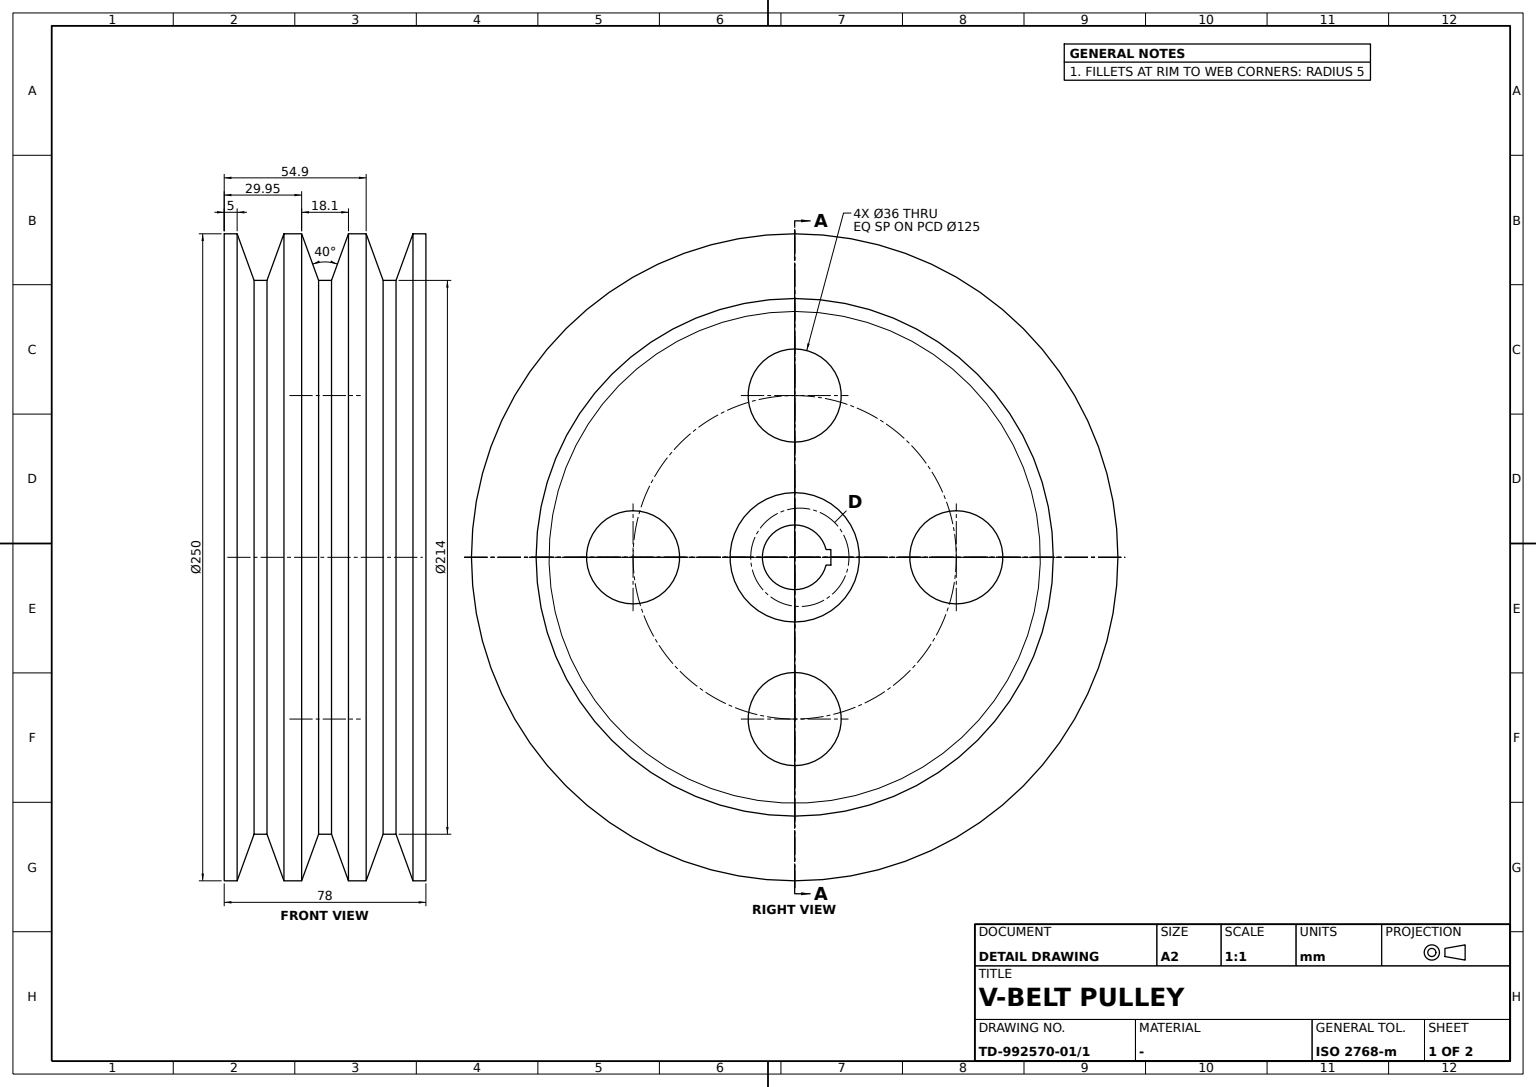
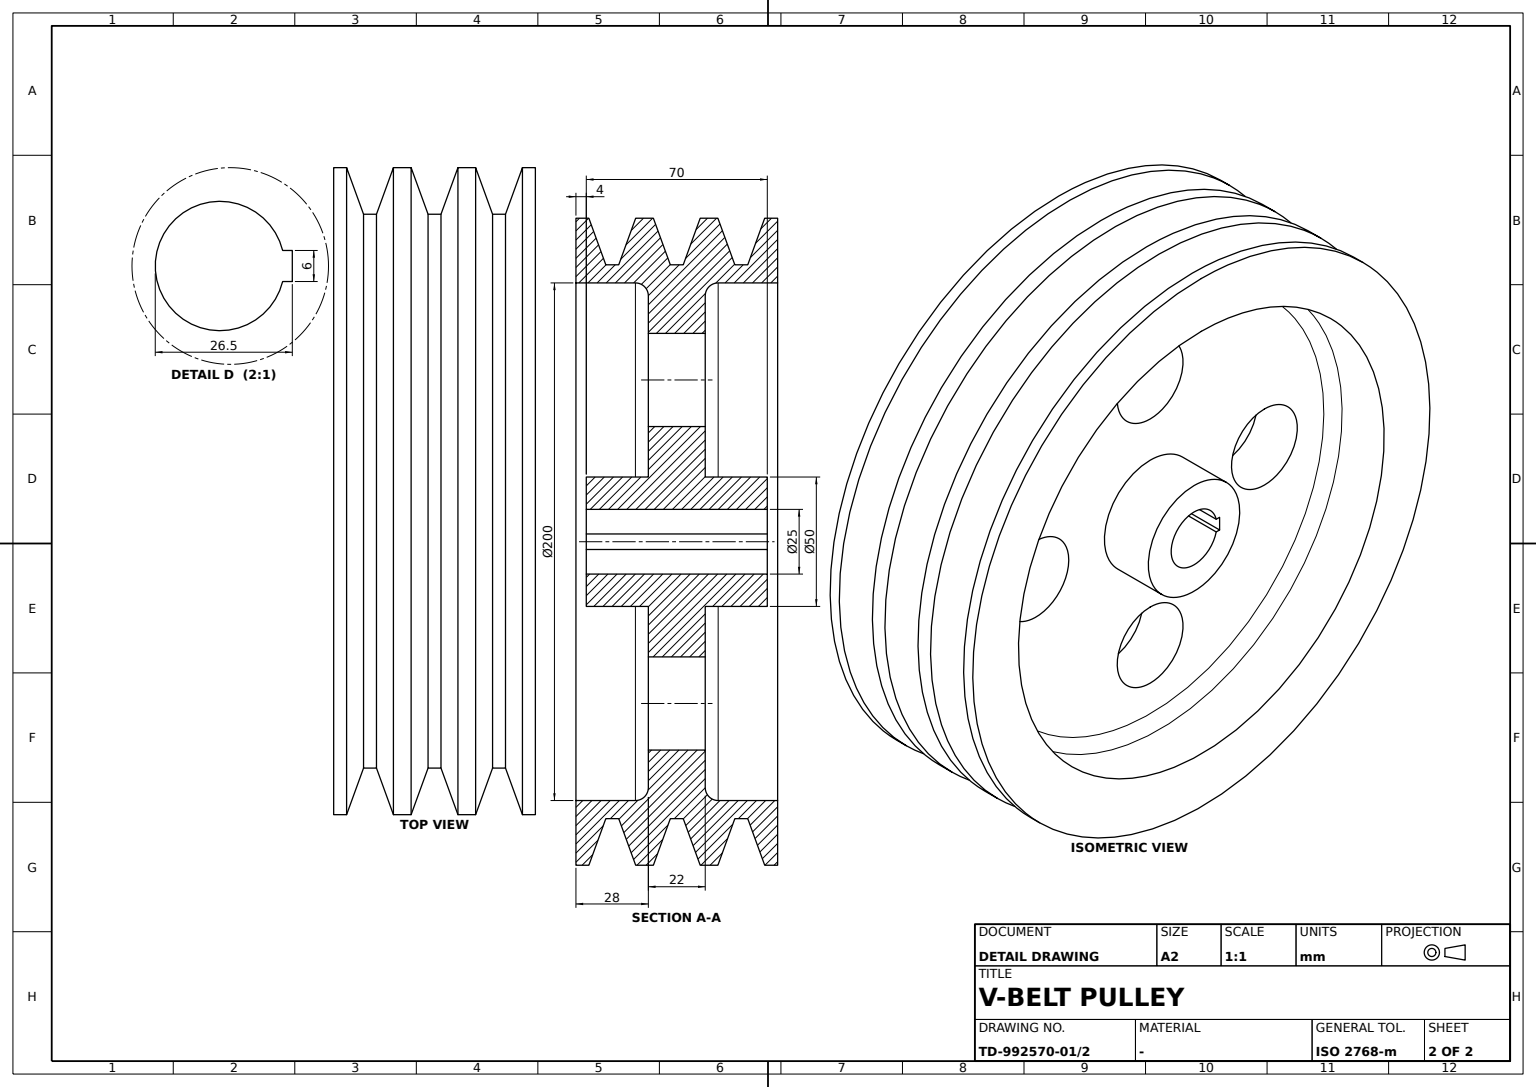
ISO-10303-21;
HEADER;
FILE_DESCRIPTION((''),'2;1');
FILE_NAME('','',(''),(''),'','','');
FILE_SCHEMA(('AUTOMOTIVE_DESIGN'));
ENDSEC;
DATA;
#1=APPLICATION_CONTEXT('');
#2=PRODUCT_CONTEXT('',#1,'mechanical');
#3=PRODUCT('','','',(#2));
#4=PRODUCT_DEFINITION_FORMATION('','',#3);
#5=PRODUCT_DEFINITION_CONTEXT('',#1,'design');
#6=PRODUCT_DEFINITION('','',#4,#5);
#7=PRODUCT_DEFINITION_SHAPE('','',#6);
#8=(LENGTH_UNIT()NAMED_UNIT(*)SI_UNIT(.MILLI.,.METRE.));
#9=(NAMED_UNIT(*)PLANE_ANGLE_UNIT()SI_UNIT($,.RADIAN.));
#10=(NAMED_UNIT(*)SI_UNIT($,.STERADIAN.)SOLID_ANGLE_UNIT());
#11=UNCERTAINTY_MEASURE_WITH_UNIT(LENGTH_MEASURE(0.005),#8,'distance_accuracy_value','');
#12=(GEOMETRIC_REPRESENTATION_CONTEXT(3)GLOBAL_UNCERTAINTY_ASSIGNED_CONTEXT((#11))GLOBAL_UNIT_ASSIGNED_CONTEXT((#8,#9,#10))REPRESENTATION_CONTEXT('',''));
#13=CARTESIAN_POINT('',(0.,27.448536,107.));
#14=VERTEX_POINT('',#13);
#15=CARTESIAN_POINT('',(0.,27.448536,0.));
#16=DIRECTION('',(0.,1.,0.));
#17=DIRECTION('',(0.,0.,1.));
#18=AXIS2_PLACEMENT_3D('',#15,#16,#17);
#19=CIRCLE('',#18,107.);
#20=EDGE_CURVE('',#14,#14,#19,.T.);
#21=ORIENTED_EDGE('',*,*,#20,.T.);
#22=EDGE_LOOP('',(#21));
#23=FACE_BOUND('',#22,.T.);
#24=CARTESIAN_POINT('',(0.,34.,125.));
#25=VERTEX_POINT('',#24);
#26=CARTESIAN_POINT('',(0.,34.,0.));
#27=AXIS2_PLACEMENT_3D('',#26,#16,#17);
#28=CIRCLE('',#27,125.);
#29=EDGE_CURVE('',#25,#25,#28,.T.);
#30=ORIENTED_EDGE('',*,*,#29,.F.);
#31=EDGE_LOOP('',(#30));
#32=FACE_BOUND('',#31,.T.);
#33=DIRECTION('',(1.,0.,0.));
#34=AXIS2_PLACEMENT_3D('',#15,#16,#33);
#35=CONICAL_SURFACE('',#34,107.,1.221730476);
#36=ADVANCED_FACE('',(#23,#32),#35,.T.);
#37=CARTESIAN_POINT('',(0.,-15.897072,125.));
#38=VERTEX_POINT('',#37);
#39=CARTESIAN_POINT('',(0.,-15.897072,0.));
#40=AXIS2_PLACEMENT_3D('',#39,#16,#17);
#41=CIRCLE('',#40,125.);
#42=EDGE_CURVE('',#38,#38,#41,.T.);
#43=ORIENTED_EDGE('',*,*,#42,.F.);
#44=EDGE_LOOP('',(#43));
#45=FACE_BOUND('',#44,.T.);
#46=CARTESIAN_POINT('',(0.,-22.448536,107.));
#47=VERTEX_POINT('',#46);
#48=CARTESIAN_POINT('',(0.,-22.448536,0.));
#49=AXIS2_PLACEMENT_3D('',#48,#16,#17);
#50=CIRCLE('',#49,107.);
#51=EDGE_CURVE('',#47,#47,#50,.T.);
#52=ORIENTED_EDGE('',*,*,#51,.T.);
#53=EDGE_LOOP('',(#52));
#54=FACE_BOUND('',#53,.T.);
#55=AXIS2_PLACEMENT_3D('',#48,#16,#33);
#56=CONICAL_SURFACE('',#55,107.,1.221730476);
#57=ADVANCED_FACE('',(#45,#54),#56,.T.);
#58=CARTESIAN_POINT('',(0.,-2.5,-107.));
#59=VERTEX_POINT('',#58);
#60=CARTESIAN_POINT('',(0.,-2.5,0.));
#61=DIRECTION('',(0.,-1.,0.));
#62=DIRECTION('',(0.,0.,-1.));
#63=AXIS2_PLACEMENT_3D('',#60,#61,#62);
#64=CIRCLE('',#63,107.);
#65=EDGE_CURVE('',#59,#59,#64,.F.);
#66=ORIENTED_EDGE('',*,*,#65,.T.);
#67=EDGE_LOOP('',(#66));
#68=FACE_BOUND('',#67,.T.);
#69=CARTESIAN_POINT('',(0.,2.5,107.));
#70=VERTEX_POINT('',#69);
#71=CARTESIAN_POINT('',(0.,2.5,0.));
#72=AXIS2_PLACEMENT_3D('',#71,#16,#17);
#73=CIRCLE('',#72,107.);
#74=EDGE_CURVE('',#70,#70,#73,.T.);
#75=ORIENTED_EDGE('',*,*,#74,.F.);
#76=EDGE_LOOP('',(#75));
#77=FACE_BOUND('',#76,.T.);
#78=CARTESIAN_POINT('',(0.,0.,0.));
#79=AXIS2_PLACEMENT_3D('',#78,#16,#33);
#80=CYLINDRICAL_SURFACE('',#79,107.);
#81=ADVANCED_FACE('',(#68,#77),#80,.T.);
#82=CARTESIAN_POINT('',(0.,39.,100.));
#83=VERTEX_POINT('',#82);
#84=CARTESIAN_POINT('',(0.,39.,0.));
#85=AXIS2_PLACEMENT_3D('',#84,#16,#17);
#86=CIRCLE('',#85,100.);
#87=EDGE_CURVE('',#83,#83,#86,.T.);
#88=ORIENTED_EDGE('',*,*,#87,.T.);
#89=EDGE_LOOP('',(#88));
#90=FACE_BOUND('',#89,.T.);
#91=CARTESIAN_POINT('',(0.,16.,100.));
#92=VERTEX_POINT('',#91);
#93=CARTESIAN_POINT('',(0.,16.,0.));
#94=AXIS2_PLACEMENT_3D('',#93,#16,#17);
#95=CIRCLE('',#94,100.);
#96=EDGE_CURVE('',#92,#92,#95,.T.);
#97=ORIENTED_EDGE('',*,*,#96,.F.);
#98=EDGE_LOOP('',(#97));
#99=FACE_BOUND('',#98,.T.);
#100=CYLINDRICAL_SURFACE('',#79,100.);
#101=ADVANCED_FACE('',(#90,#99),#100,.F.);
#102=CARTESIAN_POINT('',(0.,35.,25.));
#103=VERTEX_POINT('',#102);
#104=CARTESIAN_POINT('',(0.,35.,0.));
#105=AXIS2_PLACEMENT_3D('',#104,#16,#17);
#106=CIRCLE('',#105,25.);
#107=EDGE_CURVE('',#103,#103,#106,.T.);
#108=ORIENTED_EDGE('',*,*,#107,.F.);
#109=EDGE_LOOP('',(#108));
#110=FACE_BOUND('',#109,.T.);
#111=CARTESIAN_POINT('',(0.,11.,25.));
#112=VERTEX_POINT('',#111);
#113=CARTESIAN_POINT('',(0.,11.,0.));
#114=AXIS2_PLACEMENT_3D('',#113,#16,#17);
#115=CIRCLE('',#114,25.);
#116=EDGE_CURVE('',#112,#112,#115,.T.);
#117=ORIENTED_EDGE('',*,*,#116,.T.);
#118=EDGE_LOOP('',(#117));
#119=FACE_BOUND('',#118,.T.);
#120=CYLINDRICAL_SURFACE('',#79,25.);
#121=ADVANCED_FACE('',(#110,#119),#120,.T.);
#122=CARTESIAN_POINT('',(0.,-11.,-44.5));
#123=VERTEX_POINT('',#122);
#124=CARTESIAN_POINT('',(0.,-11.,-62.5));
#125=AXIS2_PLACEMENT_3D('',#124,#16,#17);
#126=CIRCLE('',#125,18.);
#127=EDGE_CURVE('',#123,#123,#126,.T.);
#128=ORIENTED_EDGE('',*,*,#127,.T.);
#129=EDGE_LOOP('',(#128));
#130=FACE_BOUND('',#129,.T.);
#131=CARTESIAN_POINT('',(0.,-11.,25.));
#132=VERTEX_POINT('',#131);
#133=CARTESIAN_POINT('',(0.,-11.,0.));
#134=AXIS2_PLACEMENT_3D('',#133,#16,#17);
#135=CIRCLE('',#134,25.);
#136=EDGE_CURVE('',#132,#132,#135,.T.);
#137=ORIENTED_EDGE('',*,*,#136,.T.);
#138=EDGE_LOOP('',(#137));
#139=FACE_BOUND('',#138,.T.);
#140=CARTESIAN_POINT('',(0.,-11.,95.));
#141=VERTEX_POINT('',#140);
#142=CIRCLE('',#134,95.);
#143=EDGE_CURVE('',#141,#141,#142,.T.);
#144=ORIENTED_EDGE('',*,*,#143,.F.);
#145=EDGE_LOOP('',(#144));
#146=FACE_BOUND('',#145,.T.);
#147=CARTESIAN_POINT('',(0.,-11.,80.5));
#148=VERTEX_POINT('',#147);
#149=CARTESIAN_POINT('',(0.,-11.,62.5));
#150=AXIS2_PLACEMENT_3D('',#149,#16,#17);
#151=CIRCLE('',#150,18.);
#152=EDGE_CURVE('',#148,#148,#151,.T.);
#153=ORIENTED_EDGE('',*,*,#152,.T.);
#154=EDGE_LOOP('',(#153));
#155=FACE_BOUND('',#154,.T.);
#156=CARTESIAN_POINT('',(62.5,-11.,18.));
#157=VERTEX_POINT('',#156);
#158=CARTESIAN_POINT('',(62.5,-11.,0.));
#159=AXIS2_PLACEMENT_3D('',#158,#16,#17);
#160=CIRCLE('',#159,18.);
#161=EDGE_CURVE('',#157,#157,#160,.T.);
#162=ORIENTED_EDGE('',*,*,#161,.T.);
#163=EDGE_LOOP('',(#162));
#164=FACE_BOUND('',#163,.T.);
#165=CARTESIAN_POINT('',(-62.5,-11.,18.));
#166=VERTEX_POINT('',#165);
#167=CARTESIAN_POINT('',(-62.5,-11.,0.));
#168=AXIS2_PLACEMENT_3D('',#167,#16,#17);
#169=CIRCLE('',#168,18.);
#170=EDGE_CURVE('',#166,#166,#169,.T.);
#171=ORIENTED_EDGE('',*,*,#170,.T.);
#172=EDGE_LOOP('',(#171));
#173=FACE_BOUND('',#172,.T.);
#174=CARTESIAN_POINT('',(0.,-11.,100.));
#175=AXIS2_PLACEMENT_3D('',#174,#16,#33);
#176=PLANE('',#175);
#177=ADVANCED_FACE('',(#130,#139,#146,#155,#164,#173),#176,.F.);
#178=CARTESIAN_POINT('',(0.,39.,125.));
#179=VERTEX_POINT('',#178);
#180=CIRCLE('',#85,125.);
#181=EDGE_CURVE('',#179,#179,#180,.T.);
#182=ORIENTED_EDGE('',*,*,#181,.F.);
#183=EDGE_LOOP('',(#182));
#184=FACE_BOUND('',#183,.T.);
#185=ORIENTED_EDGE('',*,*,#29,.T.);
#186=EDGE_LOOP('',(#185));
#187=FACE_BOUND('',#186,.T.);
#188=CYLINDRICAL_SURFACE('',#79,125.);
#189=ADVANCED_FACE('',(#184,#187),#188,.T.);
#190=CARTESIAN_POINT('',(-14.,35.,-3.));
#191=VERTEX_POINT('',#190);
#192=CARTESIAN_POINT('',(-14.,-35.,-3.));
#193=VERTEX_POINT('',#192);
#194=VECTOR('',#61,1000.);
#195=LINE('',#190,#194);
#196=EDGE_CURVE('',#191,#193,#195,.T.);
#197=ORIENTED_EDGE('',*,*,#196,.T.);
#198=CARTESIAN_POINT('',(-12.134661,-35.,-3.));
#199=VERTEX_POINT('',#198);
#200=VECTOR('',#33,1000.);
#201=LINE('',#192,#200);
#202=EDGE_CURVE('',#193,#199,#201,.T.);
#203=ORIENTED_EDGE('',*,*,#202,.T.);
#204=CARTESIAN_POINT('',(-12.134661,35.,-3.));
#205=VERTEX_POINT('',#204);
#206=VECTOR('',#16,1000.);
#207=LINE('',#204,#206);
#208=EDGE_CURVE('',#205,#199,#207,.F.);
#209=ORIENTED_EDGE('',*,*,#208,.F.);
#210=LINE('',#190,#200);
#211=EDGE_CURVE('',#191,#205,#210,.T.);
#212=ORIENTED_EDGE('',*,*,#211,.F.);
#213=EDGE_LOOP('',(#197,#203,#209,#212));
#214=FACE_BOUND('',#213,.T.);
#215=AXIS2_PLACEMENT_3D('',#190,#62,#33);
#216=PLANE('',#215);
#217=ADVANCED_FACE('',(#214),#216,.F.);
#218=CARTESIAN_POINT('',(0.,9.051464,125.));
#219=VERTEX_POINT('',#218);
#220=CARTESIAN_POINT('',(0.,9.051464,0.));
#221=AXIS2_PLACEMENT_3D('',#220,#16,#17);
#222=CIRCLE('',#221,125.);
#223=EDGE_CURVE('',#219,#219,#222,.T.);
#224=ORIENTED_EDGE('',*,*,#223,.T.);
#225=EDGE_LOOP('',(#224));
#226=FACE_BOUND('',#225,.T.);
#227=CARTESIAN_POINT('',(0.,15.897072,-125.));
#228=VERTEX_POINT('',#227);
#229=CARTESIAN_POINT('',(0.,15.897072,0.));
#230=AXIS2_PLACEMENT_3D('',#229,#61,#62);
#231=CIRCLE('',#230,125.);
#232=EDGE_CURVE('',#228,#228,#231,.F.);
#233=ORIENTED_EDGE('',*,*,#232,.F.);
#234=EDGE_LOOP('',(#233));
#235=FACE_BOUND('',#234,.T.);
#236=ADVANCED_FACE('',(#226,#235),#188,.T.);
#237=CARTESIAN_POINT('',(0.,11.,95.));
#238=VERTEX_POINT('',#237);
#239=CIRCLE('',#114,95.);
#240=EDGE_CURVE('',#238,#238,#239,.T.);
#241=ORIENTED_EDGE('',*,*,#240,.T.);
#242=EDGE_LOOP('',(#241));
#243=FACE_BOUND('',#242,.T.);
#244=CARTESIAN_POINT('',(0.,11.,-44.5));
#245=VERTEX_POINT('',#244);
#246=CARTESIAN_POINT('',(0.,11.,-62.5));
#247=AXIS2_PLACEMENT_3D('',#246,#16,#17);
#248=CIRCLE('',#247,18.);
#249=EDGE_CURVE('',#245,#245,#248,.T.);
#250=ORIENTED_EDGE('',*,*,#249,.F.);
#251=EDGE_LOOP('',(#250));
#252=FACE_BOUND('',#251,.T.);
#253=CARTESIAN_POINT('',(-62.5,11.,18.));
#254=VERTEX_POINT('',#253);
#255=CARTESIAN_POINT('',(-62.5,11.,0.));
#256=AXIS2_PLACEMENT_3D('',#255,#16,#17);
#257=CIRCLE('',#256,18.);
#258=EDGE_CURVE('',#254,#254,#257,.T.);
#259=ORIENTED_EDGE('',*,*,#258,.F.);
#260=EDGE_LOOP('',(#259));
#261=FACE_BOUND('',#260,.T.);
#262=CARTESIAN_POINT('',(62.5,11.,18.));
#263=VERTEX_POINT('',#262);
#264=CARTESIAN_POINT('',(62.5,11.,0.));
#265=AXIS2_PLACEMENT_3D('',#264,#16,#17);
#266=CIRCLE('',#265,18.);
#267=EDGE_CURVE('',#263,#263,#266,.T.);
#268=ORIENTED_EDGE('',*,*,#267,.F.);
#269=EDGE_LOOP('',(#268));
#270=FACE_BOUND('',#269,.T.);
#271=CARTESIAN_POINT('',(0.,11.,80.5));
#272=VERTEX_POINT('',#271);
#273=CARTESIAN_POINT('',(0.,11.,62.5));
#274=AXIS2_PLACEMENT_3D('',#273,#16,#17);
#275=CIRCLE('',#274,18.);
#276=EDGE_CURVE('',#272,#272,#275,.T.);
#277=ORIENTED_EDGE('',*,*,#276,.F.);
#278=EDGE_LOOP('',(#277));
#279=FACE_BOUND('',#278,.T.);
#280=ORIENTED_EDGE('',*,*,#116,.F.);
#281=EDGE_LOOP('',(#280));
#282=FACE_BOUND('',#281,.T.);
#283=CARTESIAN_POINT('',(0.,11.,100.));
#284=AXIS2_PLACEMENT_3D('',#283,#16,#33);
#285=PLANE('',#284);
#286=ADVANCED_FACE('',(#243,#252,#261,#270,#279,#282),#285,.T.);
#287=ORIENTED_EDGE('',*,*,#65,.F.);
#288=EDGE_LOOP('',(#287));
#289=FACE_BOUND('',#288,.T.);
#290=CARTESIAN_POINT('',(0.,-9.051464,-125.));
#291=VERTEX_POINT('',#290);
#292=CARTESIAN_POINT('',(0.,-9.051464,0.));
#293=AXIS2_PLACEMENT_3D('',#292,#61,#62);
#294=CIRCLE('',#293,125.);
#295=EDGE_CURVE('',#291,#291,#294,.F.);
#296=ORIENTED_EDGE('',*,*,#295,.T.);
#297=EDGE_LOOP('',(#296));
#298=FACE_BOUND('',#297,.T.);
#299=AXIS2_PLACEMENT_3D('',#60,#61,#33);
#300=CONICAL_SURFACE('',#299,107.,1.221730476);
#301=ADVANCED_FACE('',(#289,#298),#300,.T.);
#302=CARTESIAN_POINT('',(0.,-35.,25.));
#303=VERTEX_POINT('',#302);
#304=CARTESIAN_POINT('',(0.,-35.,0.));
#305=AXIS2_PLACEMENT_3D('',#304,#16,#17);
#306=CIRCLE('',#305,25.);
#307=EDGE_CURVE('',#303,#303,#306,.T.);
#308=ORIENTED_EDGE('',*,*,#307,.F.);
#309=EDGE_LOOP('',(#308));
#310=FACE_BOUND('',#309,.T.);
#311=CARTESIAN_POINT('',(-12.134661,-35.,3.));
#312=VERTEX_POINT('',#311);
#313=CARTESIAN_POINT('',(-14.,-35.,3.));
#314=VERTEX_POINT('',#313);
#315=DIRECTION('',(-1.,0.,0.));
#316=VECTOR('',#315,1000.);
#317=LINE('',#311,#316);
#318=EDGE_CURVE('',#312,#314,#317,.T.);
#319=ORIENTED_EDGE('',*,*,#318,.F.);
#320=CIRCLE('',#305,12.5);
#321=EDGE_CURVE('',#312,#199,#320,.T.);
#322=ORIENTED_EDGE('',*,*,#321,.T.);
#323=ORIENTED_EDGE('',*,*,#202,.F.);
#324=VECTOR('',#62,1000.);
#325=LINE('',#313,#324);
#326=EDGE_CURVE('',#314,#193,#325,.T.);
#327=ORIENTED_EDGE('',*,*,#326,.F.);
#328=EDGE_LOOP('',(#319,#322,#323,#327));
#329=FACE_BOUND('',#328,.T.);
#330=AXIS2_PLACEMENT_3D('',#302,#16,#33);
#331=PLANE('',#330);
#332=ADVANCED_FACE('',(#310,#329),#331,.F.);
#333=ORIENTED_EDGE('',*,*,#170,.F.);
#334=EDGE_LOOP('',(#333));
#335=FACE_BOUND('',#334,.T.);
#336=ORIENTED_EDGE('',*,*,#258,.T.);
#337=EDGE_LOOP('',(#336));
#338=FACE_BOUND('',#337,.T.);
#339=CARTESIAN_POINT('',(-62.5,-1.,0.));
#340=AXIS2_PLACEMENT_3D('',#339,#16,#315);
#341=CYLINDRICAL_SURFACE('',#340,18.);
#342=ADVANCED_FACE('',(#335,#338),#341,.F.);
#343=CARTESIAN_POINT('',(0.,-34.,-125.));
#344=VERTEX_POINT('',#343);
#345=CARTESIAN_POINT('',(0.,-34.,0.));
#346=AXIS2_PLACEMENT_3D('',#345,#61,#62);
#347=CIRCLE('',#346,125.);
#348=EDGE_CURVE('',#344,#344,#347,.F.);
#349=ORIENTED_EDGE('',*,*,#348,.T.);
#350=EDGE_LOOP('',(#349));
#351=FACE_BOUND('',#350,.T.);
#352=CARTESIAN_POINT('',(0.,-27.448536,-107.));
#353=VERTEX_POINT('',#352);
#354=CARTESIAN_POINT('',(0.,-27.448536,0.));
#355=AXIS2_PLACEMENT_3D('',#354,#61,#62);
#356=CIRCLE('',#355,107.);
#357=EDGE_CURVE('',#353,#353,#356,.F.);
#358=ORIENTED_EDGE('',*,*,#357,.F.);
#359=EDGE_LOOP('',(#358));
#360=FACE_BOUND('',#359,.T.);
#361=AXIS2_PLACEMENT_3D('',#354,#61,#33);
#362=CONICAL_SURFACE('',#361,107.,1.221730476);
#363=ADVANCED_FACE('',(#351,#360),#362,.T.);
#364=CARTESIAN_POINT('',(0.,22.448536,-107.));
#365=VERTEX_POINT('',#364);
#366=CARTESIAN_POINT('',(0.,22.448536,0.));
#367=AXIS2_PLACEMENT_3D('',#366,#61,#62);
#368=CIRCLE('',#367,107.);
#369=EDGE_CURVE('',#365,#365,#368,.F.);
#370=ORIENTED_EDGE('',*,*,#369,.F.);
#371=EDGE_LOOP('',(#370));
#372=FACE_BOUND('',#371,.T.);
#373=ORIENTED_EDGE('',*,*,#232,.T.);
#374=EDGE_LOOP('',(#373));
#375=FACE_BOUND('',#374,.T.);
#376=AXIS2_PLACEMENT_3D('',#366,#61,#33);
#377=CONICAL_SURFACE('',#376,107.,1.221730476);
#378=ADVANCED_FACE('',(#372,#375),#377,.T.);
#379=ORIENTED_EDGE('',*,*,#181,.T.);
#380=EDGE_LOOP('',(#379));
#381=FACE_BOUND('',#380,.T.);
#382=ORIENTED_EDGE('',*,*,#87,.F.);
#383=EDGE_LOOP('',(#382));
#384=FACE_BOUND('',#383,.T.);
#385=AXIS2_PLACEMENT_3D('',#82,#16,#33);
#386=PLANE('',#385);
#387=ADVANCED_FACE('',(#381,#384),#386,.T.);
#388=CARTESIAN_POINT('',(0.,-16.,100.));
#389=VERTEX_POINT('',#388);
#390=CARTESIAN_POINT('',(0.,-16.,0.));
#391=AXIS2_PLACEMENT_3D('',#390,#16,#17);
#392=CIRCLE('',#391,100.);
#393=EDGE_CURVE('',#389,#389,#392,.T.);
#394=ORIENTED_EDGE('',*,*,#393,.T.);
#395=EDGE_LOOP('',(#394));
#396=FACE_BOUND('',#395,.T.);
#397=CARTESIAN_POINT('',(0.,-39.,100.));
#398=VERTEX_POINT('',#397);
#399=CARTESIAN_POINT('',(0.,-39.,0.));
#400=AXIS2_PLACEMENT_3D('',#399,#16,#17);
#401=CIRCLE('',#400,100.);
#402=EDGE_CURVE('',#398,#398,#401,.T.);
#403=ORIENTED_EDGE('',*,*,#402,.F.);
#404=EDGE_LOOP('',(#403));
#405=FACE_BOUND('',#404,.T.);
#406=ADVANCED_FACE('',(#396,#405),#100,.F.);
#407=ORIENTED_EDGE('',*,*,#161,.F.);
#408=EDGE_LOOP('',(#407));
#409=FACE_BOUND('',#408,.T.);
#410=ORIENTED_EDGE('',*,*,#267,.T.);
#411=EDGE_LOOP('',(#410));
#412=FACE_BOUND('',#411,.T.);
#413=CARTESIAN_POINT('',(62.5,-1.,0.));
#414=AXIS2_PLACEMENT_3D('',#413,#16,#315);
#415=CYLINDRICAL_SURFACE('',#414,18.);
#416=ADVANCED_FACE('',(#409,#412),#415,.F.);
#417=ORIENTED_EDGE('',*,*,#393,.F.);
#418=EDGE_LOOP('',(#417));
#419=FACE_BOUND('',#418,.T.);
#420=ORIENTED_EDGE('',*,*,#143,.T.);
#421=EDGE_LOOP('',(#420));
#422=FACE_BOUND('',#421,.T.);
#423=DIRECTION('',(-0.349008533,0.,0.937119546));
#424=AXIS2_PLACEMENT_3D('',#390,#16,#423);
#425=TOROIDAL_SURFACE('',#424,95.,5.);
#426=ADVANCED_FACE('',(#419,#422),#425,.F.);
#427=ORIENTED_EDGE('',*,*,#249,.T.);
#428=EDGE_LOOP('',(#427));
#429=FACE_BOUND('',#428,.T.);
#430=ORIENTED_EDGE('',*,*,#127,.F.);
#431=EDGE_LOOP('',(#430));
#432=FACE_BOUND('',#431,.T.);
#433=CARTESIAN_POINT('',(0.,-1.,-62.5));
#434=AXIS2_PLACEMENT_3D('',#433,#16,#315);
#435=CYLINDRICAL_SURFACE('',#434,18.);
#436=ADVANCED_FACE('',(#429,#432),#435,.F.);
#437=ORIENTED_EDGE('',*,*,#348,.F.);
#438=EDGE_LOOP('',(#437));
#439=FACE_BOUND('',#438,.T.);
#440=CARTESIAN_POINT('',(0.,-39.,125.));
#441=VERTEX_POINT('',#440);
#442=CIRCLE('',#400,125.);
#443=EDGE_CURVE('',#441,#441,#442,.T.);
#444=ORIENTED_EDGE('',*,*,#443,.T.);
#445=EDGE_LOOP('',(#444));
#446=FACE_BOUND('',#445,.T.);
#447=ADVANCED_FACE('',(#439,#446),#188,.T.);
#448=ORIENTED_EDGE('',*,*,#223,.F.);
#449=EDGE_LOOP('',(#448));
#450=FACE_BOUND('',#449,.T.);
#451=ORIENTED_EDGE('',*,*,#74,.T.);
#452=EDGE_LOOP('',(#451));
#453=FACE_BOUND('',#452,.T.);
#454=AXIS2_PLACEMENT_3D('',#71,#16,#33);
#455=CONICAL_SURFACE('',#454,107.,1.221730476);
#456=ADVANCED_FACE('',(#450,#453),#455,.T.);
#457=ORIENTED_EDGE('',*,*,#196,.F.);
#458=CARTESIAN_POINT('',(-14.,35.,3.));
#459=VERTEX_POINT('',#458);
#460=LINE('',#458,#324);
#461=EDGE_CURVE('',#459,#191,#460,.T.);
#462=ORIENTED_EDGE('',*,*,#461,.F.);
#463=LINE('',#458,#194);
#464=EDGE_CURVE('',#459,#314,#463,.T.);
#465=ORIENTED_EDGE('',*,*,#464,.T.);
#466=ORIENTED_EDGE('',*,*,#326,.T.);
#467=EDGE_LOOP('',(#457,#462,#465,#466));
#468=FACE_BOUND('',#467,.T.);
#469=AXIS2_PLACEMENT_3D('',#458,#315,#62);
#470=PLANE('',#469);
#471=ADVANCED_FACE('',(#468),#470,.F.);
#472=CARTESIAN_POINT('',(-12.134661,35.,3.));
#473=VERTEX_POINT('',#472);
#474=LINE('',#472,#206);
#475=EDGE_CURVE('',#473,#312,#474,.F.);
#476=ORIENTED_EDGE('',*,*,#475,.T.);
#477=ORIENTED_EDGE('',*,*,#318,.T.);
#478=ORIENTED_EDGE('',*,*,#464,.F.);
#479=LINE('',#472,#316);
#480=EDGE_CURVE('',#473,#459,#479,.T.);
#481=ORIENTED_EDGE('',*,*,#480,.F.);
#482=EDGE_LOOP('',(#476,#477,#478,#481));
#483=FACE_BOUND('',#482,.T.);
#484=AXIS2_PLACEMENT_3D('',#472,#17,#315);
#485=PLANE('',#484);
#486=ADVANCED_FACE('',(#483),#485,.F.);
#487=ORIENTED_EDGE('',*,*,#136,.F.);
#488=EDGE_LOOP('',(#487));
#489=FACE_BOUND('',#488,.T.);
#490=ORIENTED_EDGE('',*,*,#307,.T.);
#491=EDGE_LOOP('',(#490));
#492=FACE_BOUND('',#491,.T.);
#493=ADVANCED_FACE('',(#489,#492),#120,.T.);
#494=ORIENTED_EDGE('',*,*,#42,.T.);
#495=EDGE_LOOP('',(#494));
#496=FACE_BOUND('',#495,.T.);
#497=ORIENTED_EDGE('',*,*,#295,.F.);
#498=EDGE_LOOP('',(#497));
#499=FACE_BOUND('',#498,.T.);
#500=ADVANCED_FACE('',(#496,#499),#188,.T.);
#501=ORIENTED_EDGE('',*,*,#51,.F.);
#502=EDGE_LOOP('',(#501));
#503=FACE_BOUND('',#502,.T.);
#504=ORIENTED_EDGE('',*,*,#357,.T.);
#505=EDGE_LOOP('',(#504));
#506=FACE_BOUND('',#505,.T.);
#507=ADVANCED_FACE('',(#503,#506),#80,.T.);
#508=CIRCLE('',#105,12.5);
#509=EDGE_CURVE('',#473,#205,#508,.T.);
#510=ORIENTED_EDGE('',*,*,#509,.T.);
#511=ORIENTED_EDGE('',*,*,#208,.T.);
#512=ORIENTED_EDGE('',*,*,#321,.F.);
#513=ORIENTED_EDGE('',*,*,#475,.F.);
#514=EDGE_LOOP('',(#510,#511,#512,#513));
#515=FACE_BOUND('',#514,.T.);
#516=CYLINDRICAL_SURFACE('',#79,12.5);
#517=ADVANCED_FACE('',(#515),#516,.F.);
#518=ORIENTED_EDGE('',*,*,#369,.T.);
#519=EDGE_LOOP('',(#518));
#520=FACE_BOUND('',#519,.T.);
#521=ORIENTED_EDGE('',*,*,#20,.F.);
#522=EDGE_LOOP('',(#521));
#523=FACE_BOUND('',#522,.T.);
#524=ADVANCED_FACE('',(#520,#523),#80,.T.);
#525=ORIENTED_EDGE('',*,*,#461,.T.);
#526=ORIENTED_EDGE('',*,*,#211,.T.);
#527=ORIENTED_EDGE('',*,*,#509,.F.);
#528=ORIENTED_EDGE('',*,*,#480,.T.);
#529=EDGE_LOOP('',(#525,#526,#527,#528));
#530=FACE_BOUND('',#529,.T.);
#531=ORIENTED_EDGE('',*,*,#107,.T.);
#532=EDGE_LOOP('',(#531));
#533=FACE_BOUND('',#532,.T.);
#534=AXIS2_PLACEMENT_3D('',#102,#16,#33);
#535=PLANE('',#534);
#536=ADVANCED_FACE('',(#530,#533),#535,.T.);
#537=ORIENTED_EDGE('',*,*,#240,.F.);
#538=EDGE_LOOP('',(#537));
#539=FACE_BOUND('',#538,.T.);
#540=ORIENTED_EDGE('',*,*,#96,.T.);
#541=EDGE_LOOP('',(#540));
#542=FACE_BOUND('',#541,.T.);
#543=DIRECTION('',(0.516772667,0.,-0.856122661));
#544=AXIS2_PLACEMENT_3D('',#93,#16,#543);
#545=TOROIDAL_SURFACE('',#544,95.,5.);
#546=ADVANCED_FACE('',(#539,#542),#545,.F.);
#547=ORIENTED_EDGE('',*,*,#276,.T.);
#548=EDGE_LOOP('',(#547));
#549=FACE_BOUND('',#548,.T.);
#550=ORIENTED_EDGE('',*,*,#152,.F.);
#551=EDGE_LOOP('',(#550));
#552=FACE_BOUND('',#551,.T.);
#553=CARTESIAN_POINT('',(0.,-1.,62.5));
#554=AXIS2_PLACEMENT_3D('',#553,#16,#315);
#555=CYLINDRICAL_SURFACE('',#554,18.);
#556=ADVANCED_FACE('',(#549,#552),#555,.F.);
#557=ORIENTED_EDGE('',*,*,#402,.T.);
#558=EDGE_LOOP('',(#557));
#559=FACE_BOUND('',#558,.T.);
#560=ORIENTED_EDGE('',*,*,#443,.F.);
#561=EDGE_LOOP('',(#560));
#562=FACE_BOUND('',#561,.T.);
#563=AXIS2_PLACEMENT_3D('',#440,#16,#33);
#564=PLANE('',#563);
#565=ADVANCED_FACE('',(#559,#562),#564,.F.);
#566=CLOSED_SHELL('',(#36,#57,#81,#101,#121,#177,#189,#217,#236,#286,#301,#332,#342,#363,#378,#387,#406,#416,#426,#436,#447,#456,#471,#486,#493,#500,#507,#517,#524,#536,#546,#556,#565));
#567=MANIFOLD_SOLID_BREP('',#566);
#568=ADVANCED_BREP_SHAPE_REPRESENTATION('',(#567),#12);
#569=SHAPE_DEFINITION_REPRESENTATION(#7,#568);
ENDSEC;
END-ISO-10303-21;
